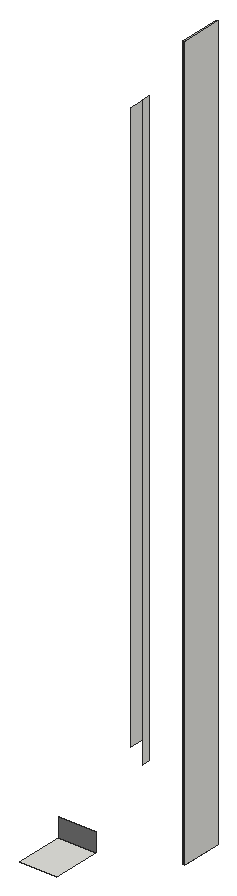
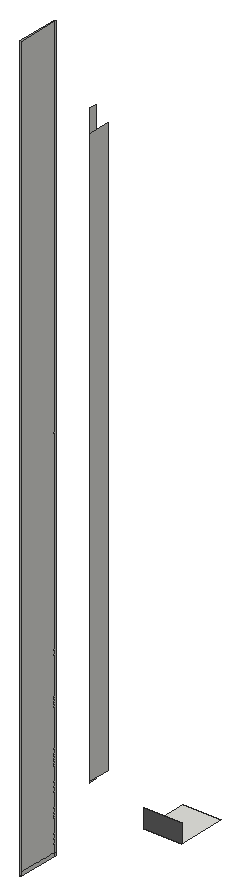
# SketchUp Ruby script. Lengths in inches.
U = 1.inch
M = Sketchup.active_model
def pt(a) = Geom::Point3d.new(a.map { |v| v * U })
def face(e, loops, mat)
  f = e.add_face(loops[0].map { |a| pt(a) })
  loops[1..].each { |l| e.add_face(l.map { |a| pt(a) }).erase! }
  f.material = f.back_material = mat if mat
  f
end
# faces: each face lists its corners as indices into pts; further lists are holes
def faces(e, pts, list, mat = nil) = list.each { |f| face(e, (f[0].is_a?(Array) ? f : [f]).map { |l| l.map { |i| pts[i] } }, mat) }
# xy, xz, yz: faces in a plane at the given z, y or x. An outline is a flat list of corners, or four numbers for a rectangle; further outlines are holes
def ring(l) = l.size == 4 ? [[l[0], l[1]], [l[2], l[1]], [l[2], l[3]], [l[0], l[3]]] : l.each_slice(2).to_a
def flat(e, list, mat, &to3) = list.each { |f| face(e, (f[0].is_a?(Array) ? f : [f]).map { |l| ring(l).map { |u, v| to3.(u, v) } }, mat) }
def xy(e, z, list, mat = nil) = flat(e, list, mat) { |x, y| [x, y, z] }
def xz(e, y, list, mat = nil) = flat(e, list, mat) { |x, z| [x, y, z] }
def yz(e, x, list, mat = nil) = flat(e, list, mat) { |y, z| [x, y, z] }
def lines(e, pts, list) = list.each { |a, b| e.add_line(pt(pts[a]), pt(pts[b])) }
# prism: a flat outline (further loops are holes) pulled along v
def prism(e, loops, v, mat = nil)
  f = face(e, loops, mat); d = Geom::Vector3d.new(v.map { |x| x * U })
  f.pushpull(f.normal.samedirection?(d) ? d.length : -d.length)
end
def box(e, o, s, mat = nil) = prism(e, [[o, [o[0] + s[0], o[1], o[2]], [o[0] + s[0], o[1] + s[1], o[2]], [o[0], o[1] + s[1], o[2]]]], [0, 0, s[2]], mat)
def at(x, y, z, deg = 0) = Geom::Transformation.translation(pt([x, y, z])) * Geom::Transformation.rotation(ORIGIN, Z_AXIS, deg.degrees)
def axes(o, x, y, z) = Geom::Transformation.new([*x, 0, *y, 0, *z, 0, *pt(o).to_a, 1])
def part(name) = M.definitions.add(name)
# library, detail: a bought-in or finely detailed component or shape, given as its bounding box
def library(name, o, s) = part(name).tap { |d| box(d.entities, o, s) }
def detail(e, o, s) = box(e.add_group.entities, o, s)
def put(e, d, t, mat = nil) = e.add_instance(d, t).tap { |i| i.material = mat if mat }
def group(e, t, mat = nil) = e.add_group.tap { |g| g.transformation = t; g.material = mat if mat }.entities
root = M.entities
M.materials.add("Generic\#4").color = [113, 113, 113]
xy(root,51,[[470.29,107.5625,470.85,108.375],[470.29,108.375,470.85,120.9375]])
xy(root,56.4375,[[443.58,75.375,455.52,90.9375]])
xz(root,90.9375,[[443.58,56.4375,455.52,62.5]],"Generic\#4")
xz(root,107.5625,[[470.29,51,470.85,288.79]])
xz(root,108.375,[[470.29,51,470.85,52.25]])
yz(root,454.83,[[106.0625,80.07,113.125,264.56]])
yz(root,458.64,[[106.0625,76.26,108.375,268.37]])
yz(root,470.29,[[107.5625,51,108.375,52.25],[108.375,51,120.9375,52.25],[107.5625,52.25,108.375,288.79],[108.375,52.25,120.9375,288.79]])
yz(root,470.85,[[107.5625,51,120.9375,288.79]])
